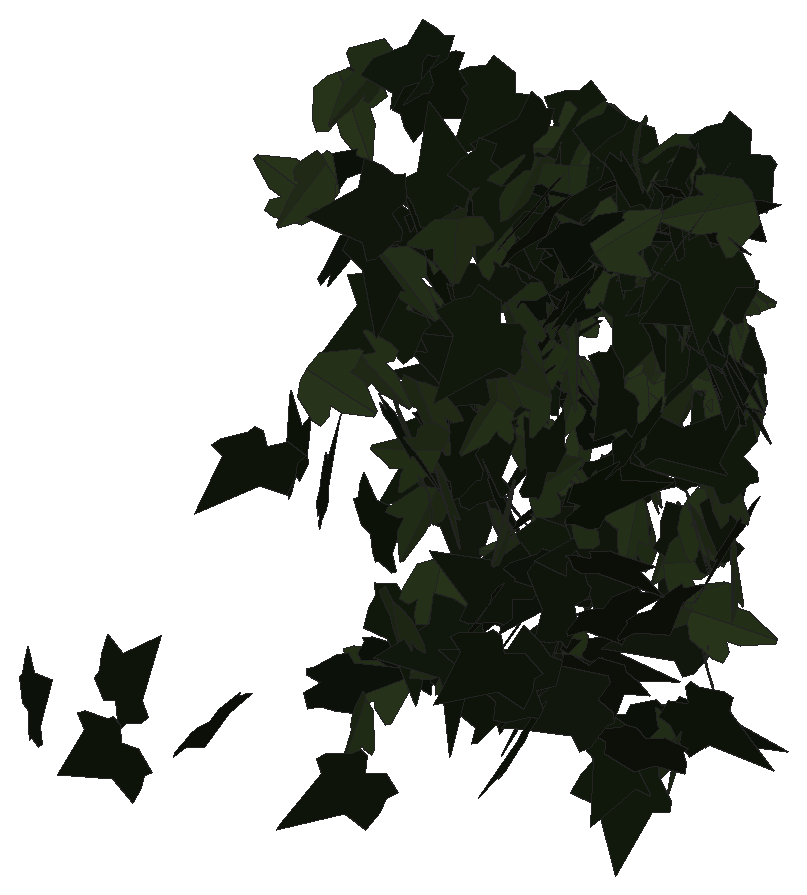
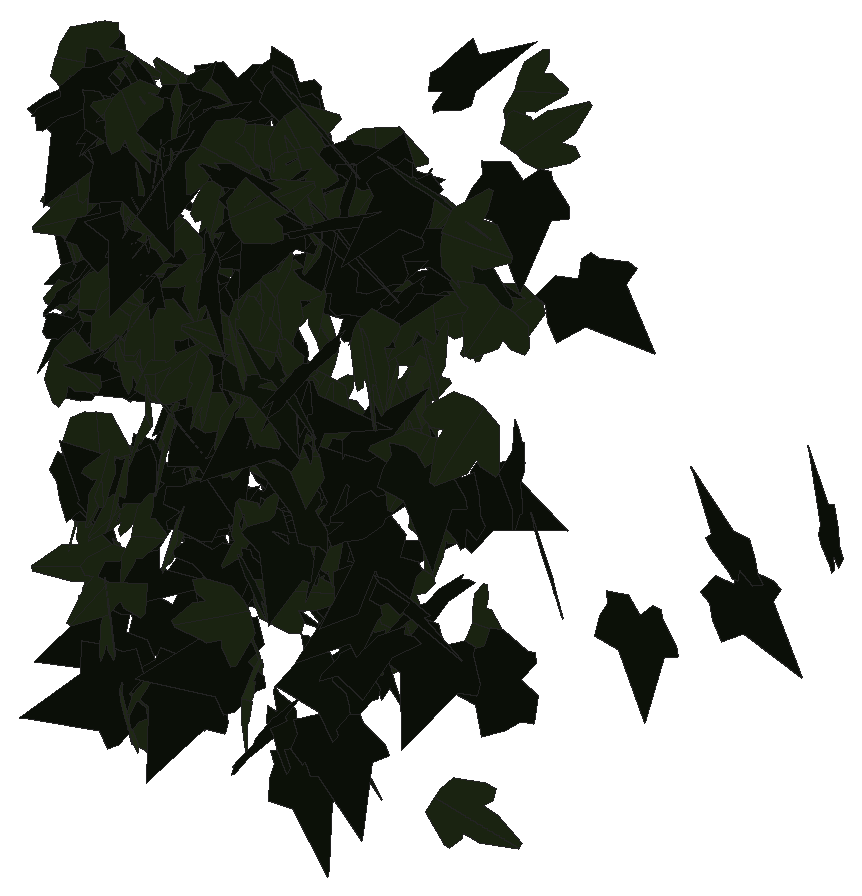
# SketchUp Ruby script. Lengths in inches.
U = 1.inch
M = Sketchup.active_model
def pt(a) = Geom::Point3d.new(a.map { |v| v * U })
def face(e, loops, mat)
  f = e.add_face(loops[0].map { |a| pt(a) })
  loops[1..].each { |l| e.add_face(l.map { |a| pt(a) }).erase! }
  f.material = f.back_material = mat if mat
  f
end
# faces: each face lists its corners as indices into pts; further lists are holes
def faces(e, pts, list, mat = nil) = list.each { |f| face(e, (f[0].is_a?(Array) ? f : [f]).map { |l| l.map { |i| pts[i] } }, mat) }
# xy, xz, yz: faces in a plane at the given z, y or x. An outline is a flat list of corners, or four numbers for a rectangle; further outlines are holes
def ring(l) = l.size == 4 ? [[l[0], l[1]], [l[2], l[1]], [l[2], l[3]], [l[0], l[3]]] : l.each_slice(2).to_a
def flat(e, list, mat, &to3) = list.each { |f| face(e, (f[0].is_a?(Array) ? f : [f]).map { |l| ring(l).map { |u, v| to3.(u, v) } }, mat) }
def xy(e, z, list, mat = nil) = flat(e, list, mat) { |x, y| [x, y, z] }
def xz(e, y, list, mat = nil) = flat(e, list, mat) { |x, z| [x, y, z] }
def yz(e, x, list, mat = nil) = flat(e, list, mat) { |y, z| [x, y, z] }
def lines(e, pts, list) = list.each { |a, b| e.add_line(pt(pts[a]), pt(pts[b])) }
# prism: a flat outline (further loops are holes) pulled along v
def prism(e, loops, v, mat = nil)
  f = face(e, loops, mat); d = Geom::Vector3d.new(v.map { |x| x * U })
  f.pushpull(f.normal.samedirection?(d) ? d.length : -d.length)
end
def box(e, o, s, mat = nil) = prism(e, [[o, [o[0] + s[0], o[1], o[2]], [o[0] + s[0], o[1] + s[1], o[2]], [o[0], o[1] + s[1], o[2]]]], [0, 0, s[2]], mat)
def at(x, y, z, deg = 0) = Geom::Transformation.translation(pt([x, y, z])) * Geom::Transformation.rotation(ORIGIN, Z_AXIS, deg.degrees)
def axes(o, x, y, z) = Geom::Transformation.new([*x, 0, *y, 0, *z, 0, *pt(o).to_a, 1])
def part(name) = M.definitions.add(name)
# library, detail: a bought-in or finely detailed component or shape, given as its bounding box
def library(name, o, s) = part(name).tap { |d| box(d.entities, o, s) }
def detail(e, o, s) = box(e.add_group.entities, o, s)
def put(e, d, t, mat = nil) = e.add_instance(d, t).tap { |i| i.material = mat if mat }
def group(e, t, mat = nil) = e.add_group.tap { |g| g.transformation = t; g.material = mat if mat }.entities
root = M.entities
M.materials.add("efeu1").color = [18, 25, 13]
M.materials.add("efeu2").color = [43, 57, 29]
c1 = part("ivyleaf_9")
p = [[1.54,2.16,1.25],[1.36,2.04,1.19],[-0.21,0.99,0.68],[-0.71,1.11,0.82],[-0.85,0.86,0.67],[-0.8,0.17,0.21],
  [-0.9,-0.01,0.1],[-0.67,-0.16,-0.02],[-0.08,-0.08,-0.05],[-0.03,-0.6,-0.4],[0.65,-0.88,-0.66],[0.83,-0.6,-0.49],
  [1.29,-0.42,-0.43],[1.8125,-0.07,-0.26],[1.21,0.44,0.15]]
faces(c1.entities,p,[[0,1,2,3,4,5,6,7,8,9,10,11,12,13,14]],"efeu1")
c2 = part("ivyleaf_10")
p = [[0,0.5,-0.03],[-0.0625,2.02,-0.43],[-0.19,2.01,-0.46],[-0.54,1.05,-0.29],[-0.52,0.625,-0.18],[-0.83,0.76,-0.28],
  [-1.16,0.64,-0.33],[-1.15,0.33,-0.24],[-0.77,-0.39,0.02],[-0.3,-0.51,0.16],[0.04,-0.48,0.23],[-0.02,2.01,-0.4375],
  [-0.06,2.01,-0.43],[0.04,-0.49,0.23],[0.67,-0.49,0.14],[1.38,0.36,-0.2],[1.375,0.51,-0.24],[0.81,0.65,-0.19],
  [0.62,0.59,-0.15],[0.6,1.09,-0.28],[0.5,1.23,-0.31]]
faces(c2.entities,p,[[0,1,2,3,4,5,6,7,8,9,10],[11,12,0,13,14,15,16,17,18,19,20]],"efeu2")
put(root,c1,axes([2.03,216.64,215.59],[-0.03567,0.11678,0.43444],[0.1332,-0.39912,0.12618],[0.44911,0.12765,-0.00292]))
put(root,c1,axes([2.93,217.38,215.04],[0.06435,0.06376,-0.4432],[-0.38914,-0.22857,-0.08796],[-0.25522,0.36458,0.02236]))
put(root,c1,axes([2.71,217.64,215.57],[-0.17026,0.19971,0.36694],[0.22935,-0.2818,0.26457],[0.37299,0.26444,0.00482]))
put(root,c1,axes([6.42,218.1,215.48],[-0.05514,0.023,-0.44864],[-0.02604,-0.43386,-0.02109],[-0.46583,0.02153,0.05429]))
put(root,c1,axes([4.34,218.66,219.4],[0.00701,0.16049,-0.42043],[-0.07443,-0.39882,-0.16581],[-0.46381,0.06643,0.02025]))
put(root,c1,axes([3.43,218.66,215],[-0.03011,0.43265,0.03692],[-0.00719,0.03515,-0.45087],[-0.46878,-0.02833,0.00455]))
put(root,c2,axes([4.91,220.02,215.02],[-0.05901,0.24453,-0.36981],[-0.00912,-0.35897,-0.25538],[-0.46599,-0.02394,0.05183]))
put(root,c2,axes([4.125,220.0625,222.8],[0.07264,0.19682,-0.39733],[-0.10976,-0.36845,-0.21601],[-0.45099,0.12138,-0.01142]))
put(root,c1,axes([5.15,220.25,222.53],[-0.14018,-0.10267,0.41838],[-0.30117,-0.29071,-0.17073],[0.3322,-0.30688,0.02177]))
put(root,c1,axes([7.08,220.21,216.59],[0.07201,0.10864,-0.43254],[-0.25576,-0.34197,-0.13238],[-0.38745,0.24593,0.00699]))
put(root,c1,axes([5.29,220.11,219.61],[0.40598,-0.17785,-0.13272],[-0.12251,0.05862,-0.43247],[0.20219,0.39263,0.00445]))
put(root,c2,axes([3.78,220.33,222.25],[0.17473,0.26285,0.31879],[-0.1918,-0.25024,0.32066],[0.39165,-0.23982,0.01481]))
put(root,c2,axes([5.63,220.49,219.02],[-0.13231,-0.08604,-0.42477],[-0.24864,-0.34113,0.14655],[-0.37601,0.25584,0.05256]))
put(root,c2,axes([7.07,220.17,218.22],[0.22463,-0.27774,0.27284],[-0.17146,0.20886,0.36086],[-0.37531,-0.26165,-0.00156]))
put(root,c2,axes([4.15,220.1,219.75],[0.11432,0.24391,0.35805],[0.14006,0.31895,-0.27648],[-0.43362,0.16733,0.00509]))
put(root,c2,axes([5.29,220.28,216.57],[-0.41649,0.17327,0.10648],[-0.09942,0.04493,-0.43968],[-0.19329,-0.39646,-0.00329]))
put(root,c2,axes([5.54,220.6,218.2],[-0.08028,-0.39282,0.17829],[-0.01658,-0.17144,-0.41548],[0.46259,-0.07432,0.01605]))
put(root,c1,axes([7.18,220.57,215.26],[-0.29588,0.31384,-0.13021],[0.08912,-0.09416,-0.43326],[-0.35387,-0.28612,-0.00024]))
put(root,c1,axes([7.23,220.66,215.96],[-0.18052,0.02803,0.41665],[-0.42288,0.08508,-0.17609],[-0.09641,-0.42568,-0.00776]))
put(root,c2,axes([4.36,220.72,219.9375],[-0.25771,0.07133,-0.37091],[0.3645,-0.11556,-0.25888],[-0.1464,-0.41326,0.00837]))
put(root,c1,axes([5.81,221.03,215.92],[-0.20675,-0.12357,0.38537],[-0.3041,-0.24236,-0.23534],[0.29239,-0.33944,0.02774]))
put(root,c2,axes([5.72,220.68,218.5],[-0.32335,0.31418,-0.03081],[0.02009,-0.02319,-0.45134],[-0.34022,-0.29997,0.00262]))
put(root,c2,axes([4.77,220.93,218.99],[-0.11167,0.01339,0.43921],[0.40029,-0.20589,0.10117],[0.21912,0.38295,0.03903]))
put(root,c2,axes([5.39,220.71,219.7],[-0.45301,0.08944,-0.07561],[0.07792,-0.01022,-0.44601],[-0.09708,-0.42558,-0.00518]))
put(root,c1,axes([6.375,220.98,220.96],[-0.42131,-0.19223,0.0101],[-0.009,-0.00505,-0.45229],[0.20768,-0.39019,0.00088]))
put(root,c2,axes([7.37,220.64,220.45],[0.10328,-0.09401,-0.43037],[-0.34125,0.26739,-0.13911],[0.30594,0.32999,-0.00988]))
put(root,c1,axes([4.41,221.08,221.34],[0.01288,-0.40976,0.15136],[0.00286,-0.14552,-0.42633],[0.46961,0.01213,-0.00156]))
put(root,c1,axes([3.81,220.53,217.6],[-0.00297,-0.0104,0.45226],[0.05373,0.43201,0.01107],[-0.46671,0.04981,-0.00161]))
put(root,c2,axes([5.47,220.5625,218.39],[0.1187,0.05224,-0.43434],[-0.25184,0.36689,-0.0161],[0.37842,0.22778,0.12553]))
put(root,c1,axes([3.81,220.59,214.87],[0.1435,0.26294,-0.33285],[0.12567,0.29889,0.30561],[0.42933,-0.17537,0.0218]))
put(root,c1,axes([4.26,221.03,217.09],[-0.03689,0.04863,0.44816],[0.22392,-0.37782,0.06143],[0.41135,0.21003,0.00675]))
put(root,c1,axes([4.68,221.13,220.53],[-0.37319,-0.18768,0.19346],[-0.17425,-0.09266,-0.40893],[0.22601,-0.38134,0.00415]))
put(root,c2,axes([4.61,221.04,221.24],[-0.38926,-0.03117,-0.25121],[0.26133,0.0033,-0.37593],[0.02995,-0.43387,0.01519]))
put(root,c1,axes([7.29,220.87,219.16],[-0.08718,0.21951,0.38145],[-0.172,0.33094,-0.24243],[-0.4284,-0.17754,0.01971]))
put(root,c1,axes([4.61,221.33,215.98],[0.00837,-0.43412,-0.02753],[0.00668,0.02658,-0.45151],[0.46968,0.00736,0.00691]))
put(root,c2,axes([5.52,221.2,221.99],[-0.29592,-0.33785,-0.00259],[0.00033,0.00296,-0.45239],[0.36489,-0.27399,-0.00169]))
put(root,c1,axes([8.05,220.96,218.04],[0.4228,0.18614,0.03777],[0.00442,0.075,-0.44561],[-0.20477,0.38594,0.06837]))
put(root,c1,axes([3.3,221.11,222.2],[0.14648,0.39839,-0.11447],[-0.03621,-0.10486,-0.43767],[-0.44491,0.1397,-0.00207]))
put(root,c1,axes([6.17,221.49,216.58],[0.06502,0.00202,0.44804],[-0.44611,-0.1233,0.06063],[0.13217,-0.41715,-0.01575]))
put(root,c2,axes([5.2,221.64,215.33],[-0.02454,0.04859,0.44895],[0.0588,-0.42854,0.05314],[0.46546,0.05669,0.01695]))
put(root,c1,axes([7.4,221.28,217.01],[-0.29965,-0.00992,-0.34827],[-0.3611,-0.01944,0.2887],[-0.023,0.43445,0.00497]))
put(root,c1,axes([7.74,221.11,218.7],[0.19844,0.1703,0.36984],[0.29023,0.233,-0.26045],[-0.3116,0.32548,-0.00706]))
put(root,c1,axes([5.69,221.54,219.7],[-0.08769,0.01378,0.44422],[-0.46055,0.02595,-0.08518],[-0.03033,-0.43401,0.00901]))
put(root,c1,axes([8.01,221.22,217.18],[0.14767,0.41271,-0.01478],[-0.00625,-0.01305,-0.45216],[-0.44594,0.13685,0.00144]))
put(root,c1,axes([6.77,221.16,222.4],[0.02456,0.40355,0.16722],[0.01401,0.1603,-0.42035],[-0.46895,0.02592,-0.0038]))
put(root,c1,axes([4.43,221.27,215.37],[0.35106,0.2793,-0.07755],[-0.0618,-0.04782,-0.4457],[-0.30603,0.33005,0.00105]))
put(root,c1,axes([5.2,221.62,215.3125],[-0.28523,0.00468,-0.35945],[0.37282,-0.01864,-0.27459],[-0.01907,-0.43458,0.0079]))
put(root,c1,axes([5.05,221.54,220.95],[0.0626,-0.36275,0.24229],[-0.04039,0.22996,0.38205],[-0.46386,-0.06898,-0.00057]))
put(root,c1,axes([7.48,221.63,215.4375],[-0.41801,0.00055,0.20648],[-0.21441,0.00356,-0.40252],[-0.00229,-0.43499,-0.00304]))
put(root,c1,axes([5.98,221.87,216.46],[-0.22324,0.04097,-0.39578],[0.2094,-0.3617,-0.15002],[-0.35641,-0.23816,0.15975]))
put(root,c1,axes([3.33,221.38,220.57],[-0.17508,0.40159,0.04252],[0.01048,-0.04017,0.45035],[0.43583,0.16229,0.00625]))
put(root,c2,axes([7.57,221.3,218.34],[0.00836,-0.00004,0.45233],[-0.18857,0.39841,0.00328],[-0.43021,-0.17463,0.00736]))
put(root,c2,axes([4.82,221.7,216.29],[0.23495,0.35339,-0.13564],[-0.07256,-0.11179,-0.43159],[-0.4003,0.22768,-0.00138]))
put(root,c1,axes([5.16,221.99,218.18],[-0.06402,-0.08846,0.43864],[-0.24835,-0.35357,-0.11073],[0.39362,-0.23747,0.00147]))
put(root,c2,axes([5.14,222,221.64],[-0.02691,-0.14106,-0.42717],[-0.06723,-0.40601,0.14894],[-0.46418,0.06699,0.0032]))
put(root,c1,axes([7.65,222.02,220],[-0.03297,-0.27715,0.34724],[-0.02843,-0.33292,-0.2899],[0.46778,-0.03977,0.00686]))
put(root,c1,axes([8.34,221.45,219.68],[-0.14393,0.38049,0.16991],[-0.08432,0.14546,-0.41855],[-0.43919,-0.15262,0.02467]))
put(root,c1,axes([4.82,221.79,220.26],[0.13103,-0.3984,-0.13067],[-0.03721,0.12085,-0.43311],[0.44962,0.1261,0.00224]))
put(root,c1,axes([6.48,221.48,222.42],[-0.05251,0.40587,0.15473],[-0.01564,0.1481,-0.42511],[-0.46659,-0.05064,-0.00316]))
put(root,c1,axes([2.61,221.48,217.24],[0.00212,0.08622,0.44342],[-0.10934,0.41475,-0.08674],[-0.4569,-0.09885,0.02282]))
put(root,c1,axes([7.3,221.66,222.46],[0.08929,0.39492,-0.16907],[-0.05385,-0.15553,-0.4193],[-0.45808,0.09526,0.01634]))
put(root,c1,axes([4.28,221.79,221.53],[-0.15137,-0.13755,-0.40367],[0.33949,0.22913,-0.2025],[0.2873,-0.34323,0.0266]))
put(root,c1,axes([6.66,221.89,217.01],[0.0459,0.22227,-0.38636],[-0.09823,-0.36037,-0.23506],[-0.45712,0.09976,0.01172]))
put(root,c1,axes([7.35,221.75,215.83],[0.35476,0.22499,-0.18223],[-0.15829,-0.09609,-0.41406],[-0.2642,0.35968,0.00338]))
put(root,c1,axes([7.54,222.23,214.49],[-0.12272,-0.38298,0.17904],[-0.03473,-0.16989,-0.41513],[0.45216,-0.117,0.01671]))
put(root,c1,axes([4.95,221.86,221.95],[-0.41996,-0.16773,0.10341],[0.09832,0.03998,0.44042],[-0.18623,0.39936,-0.00066]))
put(root,c1,axes([7.69,222.12,214.16],[-0.18417,-0.39351,-0.07568],[0.02146,0.07068,-0.44591],[0.43166,-0.1714,-0.01012]))
put(root,c1,axes([5.05,221.95,215.12],[0.38738,-0.17534,0.1796],[0.16751,-0.07594,-0.41522],[0.20636,0.39079,-0.0001]))
put(root,c1,axes([7.28,222.29,217.22],[0.02554,-0.33154,-0.29185],[0.07737,-0.27421,0.3432],[-0.46268,-0.06416,0.04129]))
put(root,c1,axes([8.11,221.91,214.93],[0.09962,0.28661,-0.32652],[-0.25415,-0.23313,-0.29323],[-0.38236,0.22964,0.10983]))
put(root,c2,axes([6.61,221.65,218.31],[0.04298,-0.02553,0.44972],[-0.12312,0.41832,0.0366],[-0.45134,-0.11654,0.03284]))
put(root,c1,axes([5.42,222.12,220.41],[-0.05114,0.05681,0.44581],[-0.46607,0.02118,-0.0525],[-0.02966,-0.43075,0.05621]))
put(root,c2,axes([7.46,221.99,222.14],[0.30119,0.0013,-0.34719],[0.36011,0.0203,0.28977],[0.01772,-0.43452,0.0125]))
put(root,c2,axes([5.8125,222.13,220.37],[-0.35186,0.18403,-0.23072],[0.19812,-0.12586,-0.38876],[-0.24012,-0.37352,0.01732]))
put(root,c2,axes([5.3125,222.36,218.85],[0.02976,0.23199,-0.38162],[-0.10673,-0.35468,-0.24092],[-0.45655,0.09804,0.03145]))
put(root,c1,axes([5.47,222.375,222.35],[-0.23469,-0.37683,0.00225],[-0.00107,-0.00193,-0.45239],[0.40698,-0.21731,0.00011]))
put(root,c2,axes([5.9,222.32,222.54],[-0.09193,-0.39216,0.17462],[-0.0403,-0.16371,-0.41734],[0.45895,-0.09293,-0.00166]))
put(root,c1,axes([7.27,221.87,218.56],[0.02052,0.18085,-0.41097],[0.06837,0.39017,0.18888],[0.46435,-0.06544,-0.00965]))
put(root,c1,axes([4.91,222.04,217.59],[-0.11309,-0.06789,0.43338],[0.43388,0.11604,0.12465],[-0.14026,0.4137,0.03616]))
put(root,c1,axes([8.2,221.97,216.9],[0.09002,0.42375,0.05415],[0.01447,0.05043,-0.44913],[-0.46087,0.08435,-0.00352]))
put(root,c1,axes([6.92,222.16,221.13],[-0.24047,0.37301,-0.02346],[0.01075,-0.02033,-0.45179],[-0.40345,-0.22288,0.00194]))
put(root,c2,axes([5.39,222.02,221.54],[-0.02715,0.31423,0.31174],[-0.04353,0.29727,-0.32761],[-0.46699,-0.04598,0.01241]))
put(root,c1,axes([5.49,222.16,214.5],[-0.28659,0.30491,0.16716],[-0.1158,0.11976,-0.42038],[-0.35379,-0.2862,0.00218]))
put(root,c2,axes([3.37,222.37,214.04],[0.22258,0.03309,-0.39692],[-0.41022,-0.0387,-0.2168],[-0.0538,0.43201,0.01098]))
put(root,c2,axes([5.38,222.28,217.07],[-0.35873,0.25011,-0.13294],[0.11283,-0.07376,-0.43241],[-0.28159,-0.34818,-0.0039]))
put(root,c1,axes([4.49,222.05,221.24],[0.06519,0.0215,0.44747],[0.41038,0.20204,-0.06594],[-0.21921,0.38463,0.00962]))
put(root,c1,axes([5.93,222.24,222.97],[-0.2968,0.28214,0.19204],[-0.16343,0.10968,-0.40852],[-0.32544,-0.3124,0.03002]))
put(root,c1,axes([5.1,222.16,222.03],[0.16541,-0.10672,-0.40862],[-0.3487,0.2239,-0.19414],[0.26788,0.35736,-0.0004]))
put(root,c2,axes([7.42,222.37,219.39],[0.28869,0.0573,0.35189],[-0.35645,-0.07459,0.28431],[0.10155,-0.42471,-0.00245]))
put(root,c2,axes([6.34,222.59,215.22],[-0.01813,-0.02781,-0.45114],[0.31324,-0.32405,0.00993],[-0.34966,-0.28886,0.03229]))
put(root,c2,axes([7.43,222.48,217.88],[0.42226,-0.17962,0.06657],[0.06326,-0.02582,-0.44747],[0.19598,0.39534,0.00102]))
put(root,c1,axes([5.8,222.73,221.07],[0.255,-0.29166,-0.22882],[0.14776,-0.17232,0.39026],[-0.36586,-0.27288,-0.00187]))
put(root,c1,axes([5.24,222.3,217.65],[0.31239,-0.06756,-0.33051],[-0.32132,0.11586,-0.30725],[0.14097,0.41381,0.03206]))
put(root,c1,axes([6.93,222.8,216.97],[-0.23243,-0.29619,0.2443],[-0.15619,-0.18523,-0.3807],[0.37721,-0.25921,-0.0071]))
put(root,c1,axes([8.63,222.66,222.87],[-0.31154,0.17951,-0.28251],[0.17812,-0.23236,-0.34183],[-0.3032,-0.32095,0.08947]))
put(root,c1,axes([8.31,222.89,221.36],[-0.12832,-0.2181,0.37141],[-0.1714,-0.32003,-0.25817],[0.41817,-0.19809,0.00815]))
put(root,c1,axes([7.6,222.59,221.9],[-0.36786,0.09123,0.26491],[-0.26931,0.0531,-0.36655],[-0.11341,-0.422,0.01114]))
put(root,c1,axes([5.99,222.54,220.27],[0.34312,0.29056,0.06463],[-0.05023,-0.04123,0.44776],[0.31695,-0.32109,0.00099]))
put(root,c1,axes([5.63,222.73,222.13],[-0.16821,-0.39401,-0.10256],[0.06049,0.08378,-0.44009],[0.43446,-0.16421,0.02156]))
put(root,c2,axes([6.22,222.75,219.9],[0.27534,-0.20472,0.29839],[0.27203,-0.14187,-0.33804],[0.26627,0.35663,0.03681]))
put(root,c2,axes([5.9375,222.63,220.57],[-0.22434,-0.38143,0.02519],[-0.01441,-0.02032,-0.45169],[0.41252,-0.20814,-0.00208]))
put(root,c1,axes([8.5,222.82,222],[-0.20801,-0.37863,-0.09737],[0.07036,0.07172,-0.44103],[0.41532,-0.20179,0.02595]))
put(root,c2,axes([5.53,222.64,218.27],[-0.22581,0.03584,-0.39496],[0.40096,-0.08036,-0.22046],[-0.09464,-0.42601,0.00836]))
put(root,c2,axes([5.39,222.49,219.17],[-0.20334,-0.30051,-0.26201],[0.15818,0.20535,-0.36859],[0.39286,-0.23822,0.0128]))
put(root,c2,axes([6.28,222.65,222.41],[-0.39394,-0.23687,0.00864],[0.0109,-0.03077,-0.45114],[0.25574,-0.36356,0.03255]))
put(root,c1,axes([6.22,222.74,220.57],[-0.22257,0.27744,-0.27472],[0.15607,-0.22149,-0.35919],[-0.38317,-0.25138,0.01327]))
put(root,c1,axes([6.22,222.79,216.91],[-0.40998,0.02716,0.21909],[-0.22871,-0.01496,-0.39486],[-0.01777,-0.43389,0.02733]))
put(root,c1,axes([5.32,222.34,215.08],[-0.19646,0.32382,-0.2355],[-0.13809,0.18763,0.38588],[0.40379,0.22172,0.01739]))
put(root,c2,axes([8.85,222.86,222.8],[0.11667,0.05968,-0.48252],[-0.4458,-0.1849,-0.13066],[-0.19403,0.46071,0.01007]))
put(root,c1,axes([5.33,222.84,219.61],[-0.00956,0.00443,-0.45228],[0.46691,-0.04731,-0.00966],[-0.05119,-0.4324,-0.00358]))
put(root,c2,axes([5.99,222.96,220.72],[-0.02469,0.22634,-0.38561],[0.00746,-0.37105,-0.23601],[-0.46909,-0.01781,0.01654]))
put(root,c2,axes([5.75,222.92,216.44],[0.02151,0.0095,0.45182],[-0.32522,-0.31324,0.02148],[0.33835,-0.30169,-0.00808]))
put(root,c1,axes([4.94,222.68,214.62],[0.22927,0.21058,-0.32857],[-0.2512,-0.21398,-0.31086],[-0.32411,0.3148,0.00849]))
put(root,c2,axes([5.53,222.7,222.33],[-0.40318,-0.01475,0.23172],[-0.24005,-0.01712,-0.38848],[0.02315,-0.43441,0.00744]))
put(root,c1,axes([6.93,223.06,222.06],[-0.09706,-0.11507,0.42616],[-0.30473,-0.29744,-0.15122],[0.34414,-0.29583,-0.01371]))
put(root,c2,axes([7.48,223.05,221.5625],[-0.06938,-0.0118,0.44727],[0.22146,-0.38311,0.02092],[0.40848,0.2057,0.06462]))
put(root,c1,axes([5.56,222.9,219.09],[-0.17253,-0.16152,-0.38581],[-0.26859,-0.2754,0.23608],[-0.34468,0.29545,0.00915]))
put(root,c2,axes([5.87,222.78,219.58],[-0.41681,-0.03195,0.20607],[-0.20141,-0.10162,-0.39481],[0.0801,-0.42175,0.07952]))
put(root,c1,axes([5.71,222.84,214.68],[-0.32087,0.22414,-0.23422],[0.19558,-0.1339,-0.38705],[-0.28197,-0.34793,-0.00193]))
put(root,c1,axes([5.01,222.65,221.63],[-0.28406,0.25148,0.24787],[-0.20074,0.15012,-0.37805],[-0.3158,-0.32163,0.01735]))
put(root,c1,axes([5.6875,222.57,221.9],[0.42796,0.16172,0.08089],[0.07973,0.02493,-0.44508],[-0.17665,0.40305,-0.00492]))
put(root,c1,axes([7.11,222.77,222.82],[0.34912,-0.27809,-0.08943],[-0.01872,0.10988,-0.43736],[0.31381,0.31594,0.07339]))
put(root,c2,axes([6.05,222.68,220.54],[-0.08468,0.40844,0.1326],[-0.08926,0.11273,-0.42841],[-0.4534,-0.09848,0.05957]))
put(root,c1,axes([5.4,222.59,217.58],[-0.13643,0.41625,-0.00026],[-0.00089,0.00001,0.4524],[0.44955,0.12633,0.00081]))
put(root,c1,axes([6.11,222.58,221.21],[0.33131,0.14157,0.28496],[0.27567,0.10038,-0.35114],[-0.18696,0.39888,-0.01277]))
put(root,c2,axes([2.63,223.18,222.59],[0.03986,-0.27415,0.41623],[0.03432,-0.41506,-0.27667],[0.49723,0.05062,-0.01427]))
put(root,c1,axes([7.99,222.85,222.84],[-0.37717,0.25728,0.03401],[-0.02822,0.01967,-0.45112],[-0.27867,-0.35021,-0.00035]))
put(root,c1,axes([7.94,223.1875,221.85],[-0.30315,-0.31704,0.10358],[-0.0307,-0.10699,-0.43751],[0.35759,-0.27796,0.05025]))
put(root,c1,axes([7.8125,222.97,222.29],[0.24633,-0.17111,0.34166],[0.30805,-0.16501,-0.29533],[0.25523,0.3643,0.02671]))
put(root,c1,axes([7.98,222.74,218.65],[-0.08859,-0.04685,0.44161],[0.45232,0.07641,0.0929],[-0.09094,0.42567,0.03192]))
put(root,c2,axes([7.56,223.23,214.24],[-0.00299,-0.07459,0.44569],[0.1222,-0.41393,-0.07417],[0.45362,0.11102,0.02292]))
put(root,c1,axes([6.36,222.74,215.17],[0.35281,0.05803,0.29257],[0.29736,0.05809,-0.34499],[-0.08837,0.42718,0.00717]))
put(root,c1,axes([3.65,222.91,223],[-0.32444,0.26478,0.17671],[-0.22381,0.01023,-0.39762],[-0.25565,-0.34498,0.12384]))
put(root,c1,axes([7.32,223.15,222.93],[-0.33512,-0.30165,-0.04589],[0.04341,0.02193,-0.44989],[0.32638,-0.31265,0.01272]))
put(root,c1,axes([8.1875,222.83,222.29],[0.11119,0.38536,-0.1805],[-0.09704,-0.15459,-0.41241],[-0.44602,0.12971,0.04473]))
put(root,c2,axes([7.91,223.05,221.43],[-0.22389,0.24584,-0.30465],[0.21563,-0.21462,-0.33426],[-0.35226,-0.28762,-0.01098]))
put(root,c2,axes([5.55,222.98,219.37],[0.19762,0.38889,-0.06981],[-0.02869,-0.06169,-0.44698],[-0.42525,0.18489,-0.00229]))
put(root,c1,axes([7.89,223.15,222.15],[-0.09745,-0.42091,-0.06512],[0.01477,0.06111,-0.44769],[0.45934,-0.09126,0.00058]))
put(root,c2,axes([6.07,223.19,219.1],[0.03862,0.30665,-0.31871],[-0.0505,-0.30297,-0.32096],[-0.46548,0.05832,0.00838]))
put(root,c1,axes([8.12,222.89,215.01],[0.00514,0.01471,-0.45211],[0.33799,0.30183,0.01419],[0.32627,-0.3129,-0.00758]))
put(root,c1,axes([7.14,222.78,214.58],[0.31292,0.32417,-0.01444],[-0.01004,-0.01031,-0.45217],[-0.35028,0.28989,0.00006]))
put(root,c2,axes([7.875,223.21,221.55],[-0.16682,-0.42529,0.20322],[-0.02585,-0.20699,-0.45441],[0.47064,-0.16212,0.04707]))
put(root,c1,axes([7.8125,223.16,222.41],[0.0553,-0.42465,-0.08241],[0.0215,0.08203,-0.4438],[0.46604,0.0466,0.03025]))
put(root,c1,axes([3.79,223.16,217.27],[-0.46721,0.04446,-0.0105],[0.00821,-0.02462,-0.45161],[-0.04855,-0.43202,0.02466]))
put(root,c1,axes([7.88,223.32,215.95],[-0.27174,-0.15053,0.3342],[-0.30154,-0.15914,-0.30489],[0.23652,-0.37582,-0.00475]))
put(root,c2,axes([7.76,223.23,219.35],[0.10899,-0.38224,0.18873],[0.05147,-0.17511,-0.41115],[0.45408,0.11159,0.0013]))
put(root,c1,axes([7.97,223.25,221.97],[-0.36438,-0.27115,-0.04493],[0.03186,0.03225,-0.45011],[0.29482,-0.33862,-0.00689]))
put(root,c1,axes([6.83,223.27,217.34],[-0.27699,-0.07473,0.35704],[-0.35515,-0.09864,-0.27782],[0.13364,-0.41703,0.00173]))
put(root,c1,axes([5.69,222.78,221.82],[0.22731,0.37378,0.0751],[0.03985,0.0621,-0.44612],[-0.40921,0.21367,-0.00173]))
put(root,c1,axes([6.67,223.37,222.75],[-0.18619,-0.3699,0.15662],[-0.07505,-0.13375,-0.42438],[0.42475,-0.18578,-0.00633]))
put(root,c2,axes([7.72,223.26,214.34],[0.20891,-0.34863,0.18092],[0.08942,-0.153,-0.41465],[0.41118,0.21041,-0.00175]))
put(root,c1,axes([8.18,223.24,220.625],[-0.43888,0.01135,-0.16097],[0.16623,-0.02609,-0.42226],[-0.02147,-0.43407,0.02117]))
put(root,c2,axes([3.39,222.95,219.27],[0.23061,0.32604,0.20094],[0.07085,0.18663,-0.40291],[-0.40313,0.21931,0.04414]))
put(root,c1,axes([5.62,222.8,217.21],[0.04093,0.39958,0.1744],[-0.00138,0.16844,-0.41711],[-0.46801,0.03445,0.01648]))
put(root,c1,axes([3.68,222.84,222.83],[0.04075,-0.06518,-0.44557],[-0.14824,0.40611,-0.07683],[0.44393,0.1416,0.01525]))
put(root,c1,axes([4.18,223.41,218.19],[-0.05237,-0.35886,-0.25067],[-0.04111,-0.23805,0.37657],[-0.46506,0.06145,-0.00506]))
put(root,c1,axes([5.22,222.98,214.15],[-0.11663,0.4195,-0.04138],[0.01129,-0.03839,-0.4505],[-0.45495,-0.10849,-0.00058]))
put(root,c1,axes([7.41,223.0625,218.62],[-0.36322,0.25057,0.12007],[-0.10537,0.06224,-0.4361],[-0.27871,-0.35009,0.0084]))
put(root,c1,axes([5.95,223.29,217.03],[-0.31403,0.05563,-0.33147],[0.32326,-0.11644,-0.30513],[-0.13267,-0.41542,0.04114]))
put(root,c1,axes([7.95,223.39,219.83],[0.06548,-0.15123,0.41947],[0.14406,-0.3807,-0.16931],[0.44235,0.14637,-0.00696]))
put(root,c1,axes([6.14,223.03,218.97],[0.45632,-0.09444,-0.04394],[-0.04167,0.021,-0.45009],[0.10367,0.42411,0.01251]))
put(root,c2,axes([6.6,223.02,221.62],[-0.36678,0.26172,0.07639],[-0.06011,0.0481,-0.44588],[-0.28736,-0.34411,-0.00423]))
put(root,c1,axes([7.2,223.24,221.32],[0.22281,-0.38272,-0.01414],[-0.003,0.01395,-0.45216],[0.41359,0.20628,0.00434]))
put(root,c1,axes([5.83,223.11,219.97],[-0.34154,0.29811,-0.01936],[0.00697,-0.02028,-0.45186],[-0.32251,-0.31614,0.01073]))
put(root,c1,axes([8.47,223.43,218.66],[-0.27829,-0.09365,0.35123],[-0.28664,-0.22161,-0.27452],[0.24719,-0.36242,0.0771]))
put(root,c1,axes([5.57,223.49,214.63],[-0.06701,-0.35259,0.25698],[-0.03493,-0.24513,-0.37221],[0.46368,-0.06942,0.00909]))
put(root,c2,axes([7.84,223.12,220.875],[0.28845,-0.29751,-0.17825],[-0.11361,0.1358,-0.41563],[0.35299,0.28683,0.01189]))
put(root,c1,axes([7.06,223.39,220.57],[-0.30693,-0.3289,-0.01744],[0.02637,0.00105,-0.45169],[0.35469,-0.28469,0.01848]))
put(root,c2,axes([7.32,222.96,218.3],[-0.24094,0.29664,0.23591],[-0.15368,0.17677,-0.38596],[-0.37288,-0.26454,0.00663]))
put(root,c1,axes([8.52,223.01,221.07],[-0.44573,0.13459,0.02902],[0.01883,-0.03633,0.45045],[0.14725,0.41206,0.03024]))
put(root,c1,axes([3.73,223.04,217.66],[0.46916,0.02212,0.00519],[0.00463,0.01381,-0.45215],[-0.02405,0.43422,0.01412]))
put(root,c2,axes([7.18,222.96,222.88],[-0.18467,0.24639,0.32769],[-0.23512,0.23014,-0.31003],[-0.36239,-0.27487,0.03416]))
put(root,c2,axes([3.99,223.3,220.74],[0.10658,-0.48455,0.06205],[0.02434,-0.05816,-0.49601],[0.4879,0.10875,0.01119]))
put(root,c1,axes([7.99,223.1,222.5],[0.20951,-0.33723,-0.30395],[-0.11895,0.28228,-0.39518],[0.43813,0.2379,0.03805]))
put(root,c1,axes([5.65,222.9,218.95],[0.3022,0.2753,0.19495],[0.14689,0.12903,-0.40823],[-0.32835,0.3111,-0.0032]))
put(root,c1,axes([7.75,223.39,221.98],[-0.44473,-0.11628,0.08147],[-0.08415,-0.01226,-0.4449],[0.12588,-0.41899,-0.00959]))
put(root,c2,axes([6.55,223.16,220.86],[0.14174,0.4132,0.03704],[0.0108,0.03419,-0.45088],[-0.44778,0.13162,0.00085]))
put(root,c2,axes([8.08,223.24,220.1875],[0.18047,0.03822,0.46473],[-0.45153,-0.11007,0.1844],[0.1164,-0.48623,-0.00522]))
put(root,c1,axes([6.29,223.38,217.01],[-0.34422,-0.23942,-0.18108],[0.16806,0.08216,-0.41373],[0.27199,-0.35377,0.02647]))
put(root,c2,axes([8.38,223.46,216.99],[-0.08628,0.17951,-0.40362],[0.14697,-0.36361,-0.20404],[-0.4378,-0.15744,0.01104]))
put(root,c1,axes([7.87,223.51,220.61],[-0.27747,-0.34883,0.04076],[0.01429,-0.05815,-0.44813],[0.37884,-0.2533,0.04675]))
put(root,c2,axes([7.89,222.9,217.07],[-0.02228,0.11858,0.43474],[-0.07117,0.41279,-0.12517],[-0.46384,-0.06903,-0.00168]))
put(root,c2,axes([7.12,223.39,219.06],[0.02964,0.33038,0.29291],[-0.12537,-0.26635,0.33669],[0.45179,-0.09558,0.07421]))
put(root,c1,axes([8.2,223.43,219.68],[0.01361,-0.00085,0.45221],[0.23011,-0.37918,-0.00719],[0.40936,0.21318,-0.01099]))
put(root,c1,axes([5.83,223.08,219.6],[-0.10321,0.42059,0.05878],[-0.16792,0.01921,-0.42204],[-0.42645,-0.10935,0.15196]))
put(root,c2,axes([8.3125,223.19,221.07],[0.38274,0.21453,0.138],[0.10102,0.10074,-0.42921],[-0.25301,0.36476,0.03738]))
put(root,c1,axes([8.17,223.33,220.56],[0.31112,-0.32359,0.04064],[0.02955,-0.02795,-0.45057],[0.35078,0.28936,0.00192]))
put(root,c1,axes([6.92,222.99,222.5],[0.11934,0.41247,0.08626],[0.02207,0.08039,-0.4441],[-0.45385,0.11237,0.00109]))
put(root,c2,axes([8.27,223.22,221.12],[0.44784,0.05686,0.12324],[0.1072,0.12161,-0.42191],[-0.09305,0.41377,0.10707]))
put(root,c2,axes([8.03,223.21,221.9],[-0.20744,0.39029,0.00282],[-0.00334,0.0015,-0.45239],[-0.42151,-0.19209,0.0022]))
put(root,c2,axes([6.57,223.26,219.28],[-0.32939,0.29296,-0.10597],[0.07419,-0.07556,-0.43976],[-0.32667,-0.31256,0.00698]))
put(root,c1,axes([3.88,223.4375,216.5],[-0.07781,-0.42004,-0.09067],[0.01631,0.08586,-0.44322],[0.46302,-0.07361,0.00037]))
put(root,c1,axes([5.6,223.25,222.1],[0.17136,-0.39378,-0.25607],[-0.01241,0.26869,-0.42149],[0.46955,0.15081,0.08231]))
put(root,c1,axes([3.25,223.07,219.07],[-0.00776,0.43314,0.04116],[-0.04972,0.0386,-0.44806],[-0.4671,-0.01131,0.04701]))
put(root,c2,axes([7.58,223.32,221.92],[0.44465,0.14008,-0.01023],[-0.00925,-0.00535,-0.45228],[-0.15137,0.41179,-0.00239]))
put(root,c2,axes([5.86,223.47,220.25],[0.23436,-0.39499,0.19763],[0.13741,-0.14741,-0.45759],[0.41975,0.26879,0.03946]))
put(root,c1,axes([6.42,223.18,218.68],[0.18571,0.26265,-0.31317],[-0.29754,-0.15951,-0.3083],[-0.31256,0.3079,0.10743]))
put(root,c2,axes([4.01,223.27,220.64],[0.29571,-0.37687,-0.14325],[-0.04364,0.14669,-0.476],[0.40081,0.29403,0.05386]))
put(root,c2,axes([8.22,223.23,221.58],[-0.01944,-0.40496,-0.16413],[-0.00845,0.15823,-0.42133],[0.46932,-0.01392,-0.01439]))
put(root,c2,axes([6,223.29,219.01],[-0.46511,-0.05864,-0.01868],[0.02396,-0.03019,-0.45072],[0.06175,-0.42997,0.03419]))
put(root,c1,axes([7.36,223.42,220.7],[0.05727,-0.06874,-0.49193],[0.48535,0.11305,0.04071],[0.10563,-0.48218,0.07967]))
put(root,c2,axes([1.92,223.33,221.87],[0.40637,0.07731,0.28086],[0.27664,0.04859,-0.41365],[-0.09126,0.49159,-0.00328]))
put(root,c2,axes([7.91,223.24,217.64],[-0.36777,0.26252,0.06859],[-0.05828,0.03802,-0.44716],[-0.28646,-0.34477,0.00292]))
put(root,c1,axes([7.83,223.62,221.3],[-0.02211,-0.00187,-0.45189],[-0.01476,-0.43478,0.00262],[-0.46905,0.01377,0.02122]))
put(root,c2,axes([8.33,223.38,219.85],[0.4635,0.05487,-0.04683],[-0.04892,-0.00075,-0.44994],[-0.05902,0.43152,0.00517]))
put(root,c2,axes([6.93,223.44,216.82],[-0.23178,0.34614,0.15895],[0.08321,-0.13205,0.42354],[0.40008,0.22799,0.004]))
put(root,c2,axes([6.97,223.35,221.23],[-0.36859,-0.07946,-0.26806],[0.2886,-0.04315,-0.35414],[0.03957,-0.4255,0.08598]))
put(root,c2,axes([6,223.1,214.93],[-0.07279,0.18678,-0.40252],[-0.18298,0.34849,0.20559],[0.42653,0.18138,0.0195]))
put(root,c1,axes([8.09,223.21,222.52],[-0.19567,0.39255,0.04988],[-0.00939,0.04879,-0.44945],[-0.42701,-0.18096,-0.01298]))
put(root,c1,axes([6.96,223.37,222.23],[0.29028,-0.37434,-0.16001],[-0.10127,0.12394,-0.47369],[0.39431,0.30742,-0.00386]))
put(root,c2,axes([7.38,223.2,222.32],[-0.31147,0.23887,0.23019],[-0.18642,0.13858,-0.38945],[-0.29824,-0.3361,0.00302]))
put(root,c2,axes([6.2,223.58,222.77],[0.11991,0.26408,-0.34045],[-0.17717,-0.28456,-0.29661],[-0.41826,0.19624,0.02804]))
put(root,c2,axes([7.59,223.18,222.59],[0.17954,0.30086,0.27726],[0.12931,0.23834,-0.35738],[-0.41444,0.2047,0.00861]))
put(root,c2,axes([2.33,223.33,220.18],[-0.46188,0.03528,-0.18821],[0.18802,-0.00949,-0.4632],[-0.03625,-0.49866,-0.0045]))
put(root,c2,axes([5.52,223.68,222.16],[0.03378,0.09956,0.43919],[-0.0836,-0.41532,0.10779],[0.46107,-0.0826,-0.01263]))
put(root,c2,axes([7.8,223.48,220.3],[-0.31528,-0.28291,0.16101],[-0.1098,-0.11744,-0.42257],[0.33054,-0.30886,0.0132]))
put(root,c1,axes([7.29,223.37,220.22],[0.29614,-0.30396,-0.15302],[-0.07457,0.13507,-0.424],[0.35701,0.28034,0.03837]))
put(root,c2,axes([5.54,223.125,220.77],[-0.0289,0.26836,-0.35496],[-0.0439,0.3389,0.28045],[0.46685,0.04848,0.0044]))
put(root,c1,axes([8.19,223.65,220.29],[-0.00879,-0.42993,0.06838],[-0.01436,-0.06549,-0.44703],[0.4695,-0.01005,-0.01239]))
put(root,c2,axes([8.16,223.15,221.04],[0.11429,-0.01275,0.43861],[0.21318,0.38579,-0.03938],[-0.40275,0.20058,0.10362]))
put(root,c2,axes([7.91,223.22,217.65],[-0.02555,0.38305,0.21299],[-0.01007,0.2046,-0.39912],[-0.469,-0.02526,-0.00303]))
put(root,c2,axes([8.08,223.27,216.16],[0.05866,0.04851,0.44601],[0.37003,0.25801,-0.07548],[-0.28346,0.34685,-0.00623]))
put(root,c1,axes([4.76,223.47,220.21],[0.19174,-0.4329,-0.16072],[-0.03993,0.15783,-0.47275],[0.46005,0.19412,0.02595]))
put(root,c2,axes([7.48,223.5625,222.89],[-0.09094,-0.40734,0.13242],[-0.01987,-0.1262,-0.43252],[0.46049,-0.08589,0.00748]))
put(root,c2,axes([7.65,223.41,219.67],[-0.06986,-0.03738,0.49368],[0.4812,0.11216,0.07658],[-0.11647,0.48582,0.0203]))
put(root,c2,axes([7.1875,223.4375,219.95],[-0.13548,-0.41426,-0.04504],[0.02066,0.03945,-0.4501],[0.44937,-0.12671,0.00711]))
put(root,c1,axes([7.87,223.24,217.13],[-0.1514,-0.07739,0.42063],[0.39438,0.17411,0.16628],[-0.20555,0.39105,0.00921]))
put(root,c2,axes([7.27,223.7,217.05],[0.01051,0.22401,-0.38767],[-0.01953,-0.37232,-0.23319],[-0.46928,0.02052,0.00102]))
put(root,c1,axes([8.41,223.52,217.57],[-0.25584,0.2752,-0.2491],[0.16752,-0.18252,-0.37764],[-0.35664,-0.28315,0.00131]))
put(root,c1,axes([8.32,223.36,220],[0.37583,-0.18075,-0.19583],[-0.18387,0.08069,-0.40777],[0.21368,0.38735,-0.00644]))
put(root,c2,axes([7.19,223.65,218.72],[-0.07904,0.26436,-0.35112],[0.08864,-0.32753,-0.28522],[-0.45454,-0.10984,0.00544]))
put(root,c2,axes([5.97,223.46,216.29],[-0.23138,0.03767,-0.39178],[0.40011,-0.06829,-0.22622],[-0.08421,-0.42795,0.00161]))
put(root,c2,axes([7.76,223.42,221.96],[-0.43117,0.14718,0.09405],[-0.11658,-0.03477,-0.43675],[-0.14565,-0.40787,0.07117]))
put(root,c2,axes([5.6875,223.31,220.07],[-0.07537,-0.05373,0.44303],[0.3608,0.26432,0.09159],[-0.2913,0.34128,-0.00119]))
put(root,c1,axes([3.92,223.4,217.15],[0.44644,-0.1344,-0.01764],[-0.01802,0.00352,-0.45205],[0.14519,0.4137,-0.00188]))
put(root,c1,axes([8.28,223.85,222.9],[-0.18659,-0.41006,0.21688],[-0.09788,-0.1937,-0.45044],[0.45344,-0.21055,-0.00799]))
put(root,c2,axes([8.13,223.43,218.07],[-0.44068,0.03196,0.15324],[-0.15976,-0.00259,-0.42543],[-0.03151,-0.43382,0.01383]))
put(root,c2,axes([7.46,223.625,220.43],[0.18407,0.32007,-0.24989],[-0.1207,-0.21271,-0.37712],[-0.41504,0.20381,-0.00116]))
put(root,c2,axes([8.32,223.75,219.16],[-0.08872,-0.29651,0.3198],[0.07766,-0.31827,-0.29919],[0.45476,-0.0035,0.11348]))
put(root,c1,axes([7.41,223.25,221.24],[0.27596,0.352,-0.00565],[-0.00327,-0.00452,-0.45236],[-0.38019,0.25554,-0.00021]))
put(root,c1,axes([6.49,223.32,221.03],[0.07625,0.02539,-0.44562],[-0.46214,0.03827,-0.07097],[0.03641,0.43257,0.03244]))
put(root,c1,axes([8.27,223.23,222.36],[0.31089,0.3238,0.04042],[0.00419,0.04844,-0.44957],[-0.35219,0.28641,0.03034]))
put(root,c1,axes([7.74,223.33,214.49],[0.38403,0.04517,0.25632],[0.26301,0.0384,-0.37272],[-0.06369,0.43094,0.00635]))
put(root,c1,axes([4.34,223.84,222.45],[-0.3255,-0.27913,0.14883],[0.00174,-0.19983,-0.40183],[0.33876,-0.26717,0.14507]))
put(root,c2,axes([5.8,223.26,217.42],[0.06546,0.33827,-0.27736],[0.00764,0.2685,0.35586],[0.46515,-0.05201,0.03318]))
put(root,c2,axes([7.82,223.3,216.18],[-0.17563,-0.22457,-0.34859],[0.20574,0.27583,-0.28831],[0.38411,-0.25042,-0.00496]))
put(root,c1,axes([7.4375,223.51,222.22],[0.05833,0.33287,-0.28577],[-0.07803,-0.26605,-0.34995],[-0.45959,0.08742,0.02314]))
put(root,c2,axes([8.06,223.3,215.53],[-0.03333,0.02235,0.45066],[-0.38713,0.24349,-0.03962],[-0.26407,-0.35978,0.00119]))
put(root,c2,axes([7.54,223.7,220.15],[0.15394,0.28363,-0.30932],[-0.19421,-0.24003,-0.32768],[-0.39912,0.22619,0.04014]))
put(root,c1,axes([5.85,223.72,222.62],[-0.46301,-0.06537,0.03538],[-0.02701,-0.05984,-0.44734],[0.07486,-0.42588,0.05742]))
put(root,c1,axes([8.16,223.73,219.74],[-0.37862,-0.25262,-0.05209],[0.04549,0.02721,-0.44938],[0.27439,-0.35308,0.00263]))
